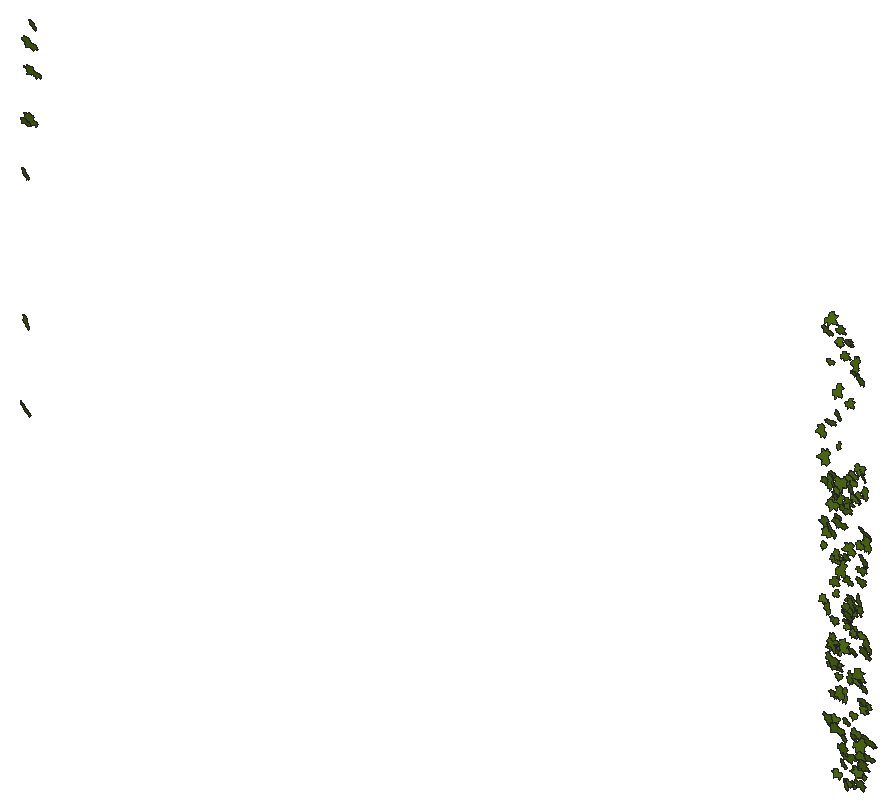
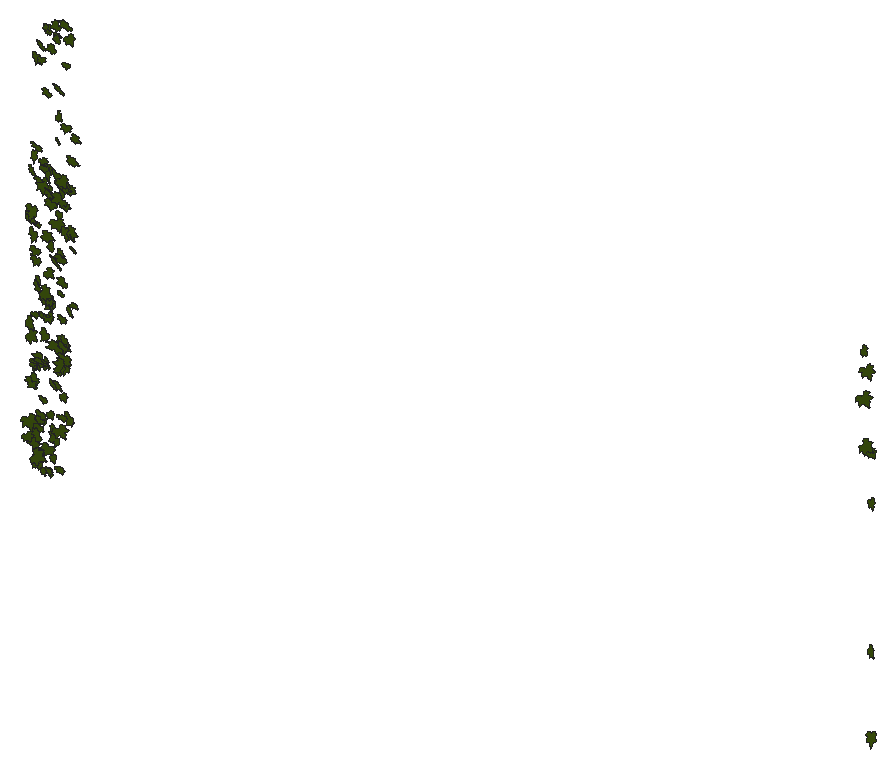
# SketchUp Ruby script. Lengths in inches.
U = 1.inch
M = Sketchup.active_model
def pt(a) = Geom::Point3d.new(a.map { |v| v * U })
def face(e, loops, mat)
  f = e.add_face(loops[0].map { |a| pt(a) })
  loops[1..].each { |l| e.add_face(l.map { |a| pt(a) }).erase! }
  f.material = f.back_material = mat if mat
  f
end
# faces: each face lists its corners as indices into pts; further lists are holes
def faces(e, pts, list, mat = nil) = list.each { |f| face(e, (f[0].is_a?(Array) ? f : [f]).map { |l| l.map { |i| pts[i] } }, mat) }
# xy, xz, yz: faces in a plane at the given z, y or x. An outline is a flat list of corners, or four numbers for a rectangle; further outlines are holes
def ring(l) = l.size == 4 ? [[l[0], l[1]], [l[2], l[1]], [l[2], l[3]], [l[0], l[3]]] : l.each_slice(2).to_a
def flat(e, list, mat, &to3) = list.each { |f| face(e, (f[0].is_a?(Array) ? f : [f]).map { |l| ring(l).map { |u, v| to3.(u, v) } }, mat) }
def xy(e, z, list, mat = nil) = flat(e, list, mat) { |x, y| [x, y, z] }
def xz(e, y, list, mat = nil) = flat(e, list, mat) { |x, z| [x, y, z] }
def yz(e, x, list, mat = nil) = flat(e, list, mat) { |y, z| [x, y, z] }
def lines(e, pts, list) = list.each { |a, b| e.add_line(pt(pts[a]), pt(pts[b])) }
# prism: a flat outline (further loops are holes) pulled along v
def prism(e, loops, v, mat = nil)
  f = face(e, loops, mat); d = Geom::Vector3d.new(v.map { |x| x * U })
  f.pushpull(f.normal.samedirection?(d) ? d.length : -d.length)
end
def box(e, o, s, mat = nil) = prism(e, [[o, [o[0] + s[0], o[1], o[2]], [o[0] + s[0], o[1] + s[1], o[2]], [o[0], o[1] + s[1], o[2]]]], [0, 0, s[2]], mat)
def at(x, y, z, deg = 0) = Geom::Transformation.translation(pt([x, y, z])) * Geom::Transformation.rotation(ORIGIN, Z_AXIS, deg.degrees)
def axes(o, x, y, z) = Geom::Transformation.new([*x, 0, *y, 0, *z, 0, *pt(o).to_a, 1])
def part(name) = M.definitions.add(name)
# library, detail: a bought-in or finely detailed component or shape, given as its bounding box
def library(name, o, s) = part(name).tap { |d| box(d.entities, o, s) }
def detail(e, o, s) = box(e.add_group.entities, o, s)
def put(e, d, t, mat = nil) = e.add_instance(d, t).tap { |i| i.material = mat if mat }
def group(e, t, mat = nil) = e.add_group.tap { |g| g.transformation = t; g.material = mat if mat }.entities
root = M.entities
M.materials.add("[Vegetation Blur 03]").color = [83, 114, 18]
c1 = part("ivy")
xy(c1.entities,0,[[0.782,0,0.786,0,0.787,0.005,0.789,0.009,0.821,0.072,0.875,0.147,1.001,0.272,1.073,0.331,1.137,0.363,1.178,0.379,1.223,0.384,1.272,0.383,1.311,0.374,1.36,0.355,1.399,0.334,1.491,0.285,1.541,0.244,1.583,0.199,1.617,0.15,1.64,0.128,1.662,0.115,1.717,0.105,1.745,0.093,1.784,0.054,1.819,0.057,1.854,0.064,1.882,0.075,1.896,0.074,1.91,0.071,1.937,0.063,1.964,0.053,1.99,0.038,2.016,0.015,2.034,0.002,2.04,0,2.038,0.003,2.036,0.007,2.033,0.038,2.036,0.068,2.045,0.1,2.055,0.116,2.064,0.123,2.077,0.129,2.088,0.129,2.106,0.132,2.118,0.13,2.179,0.132,2.207,0.133,2.225,0.133,2.242,0.138,2.22,0.162,2.207,0.186,2.206,0.213,2.212,0.236,2.228,0.262,2.247,0.274,2.298,0.283,2.355,0.294,2.37,0.296,2.376,0.295,2.377,0.3,2.377,0.303,2.385,0.329,2.411,0.37,2.426,0.392,2.449,0.407,2.511,0.426,2.561,0.444,2.619,0.466,2.589,0.469,2.561,0.476,2.501,0.5,2.449,0.516,2.424,0.523,2.401,0.535,2.377,0.556,2.372,0.568,2.36,0.575,2.268,0.586,2.225,0.592,2.207,0.599,2.194,0.61,2.143,0.65,2.13,0.664,2.122,0.682,2.123,0.7,2.13,0.719,2.148,0.75,2.17,0.781,2.195,0.807,2.221,0.828,2.284,0.874,2.291,0.88,2.288,0.887,2.276,0.9,2.267,0.916,2.265,0.933,2.273,0.967,2.292,1.002,2.313,1.03,2.334,1.054,2.348,1.067,2.358,1.074,2.363,1.076,2.362,1.081,2.35,1.094,2.347,1.11,2.35,1.143,2.359,1.18,2.385,1.254,2.415,1.324,2.448,1.393,2.45,1.4,2.446,1.398,2.44,1.394,2.427,1.383,2.402,1.36,2.376,1.339,2.345,1.324,2.305,1.309,2.282,1.303,2.273,1.306,2.245,1.294,2.212,1.287,2.187,1.291,2.163,1.301,2.142,1.316,2.134,1.327,2.124,1.325,2.09,1.292,2.053,1.259,2.014,1.234,1.973,1.215,1.954,1.21,1.931,1.208,1.909,1.212,1.893,1.22,1.879,1.233,1.872,1.248,1.867,1.281,1.864,1.319,1.821,1.258,1.773,1.197,1.726,1.141,1.698,1.121,1.679,1.116,1.666,1.117,1.647,1.122,1.632,1.129,1.62,1.141,1.617,1.154,1.617,1.219,1.621,1.254,1.623,1.268,1.623,1.281,1.618,1.314,1.606,1.346,1.603,1.375,1.607,1.403,1.603,1.467,1.599,1.499,1.605,1.525,1.614,1.552,1.629,1.577,1.635,1.589,1.629,1.587,1.618,1.582,1.596,1.566,1.581,1.556,1.568,1.552,1.557,1.55,1.545,1.553,1.531,1.562,1.522,1.572,1.504,1.591,1.486,1.611,1.474,1.631,1.457,1.666,1.455,1.684,1.457,1.698,1.452,1.715,1.444,1.728,1.424,1.754,1.419,1.772,1.423,1.786,1.434,1.819,1.444,1.848,1.446,1.855,1.44,1.861,1.43,1.867,1.386,1.904,1.349,1.948,1.326,1.973,1.31,1.995,1.288,2.048,1.284,2.153,1.287,2.254,1.284,2.255,1.282,2.253,1.278,2.247,1.274,2.237,1.266,2.216,1.226,2.125,1.208,2.076,1.184,2.033,1.155,1.984,1.135,1.942,1.111,1.899,1.083,1.861,1.053,1.85,1.059,1.83,1.061,1.809,1.056,1.79,1.049,1.767,1.04,1.749,1.018,1.733,0.994,1.726,0.942,1.734,0.95,1.6875,0.944,1.645,0.932,1.608,0.911,1.585,0.881,1.58,0.854,1.582,0.828,1.588,0.785,1.618,0.773,1.625,0.775,1.614,0.779,1.598,0.796,1.502,0.818,1.402,0.861,1.283,0.882,1.224,0.894,1.174,0.892,1.148,0.886,1.123,0.881,1.107,0.872,1.099,0.849,1.094,0.818,1.092,0.789,1.098,0.762,1.107,0.753,1.113,0.721,1.139,0.698,1.163,0.678,1.194,0.665,1.224,0.628,1.28,0.612,1.312,0.606,1.327,0.606,1.314,0.599,1.282,0.594,1.267,0.581,1.256,0.544,1.245,0.512,1.244,0.473,1.249,0.444,1.256,0.382,1.288,0.339,1.306,0.324,1.316,0.317,1.324,0.309,1.326,0.27,1.314,0.227,1.313,0.185,1.3125,0.152,1.317,0.122,1.328,0.092,1.345,0.073,1.353,0.079,1.338,0.092,1.308,0.117,1.249,0.13,1.215,0.139,1.164,0.147,1.148,0.157,1.136,0.163,1.122,0.174,1.086,0.177,1.067,0.182,1.054,0.186,1.043,0.191,1.038,0.211,1.028,0.237,1.005,0.25,0.974,0.253,0.96,0.25,0.944,0.242,0.914,0.243,0.906,0.249,0.902,0.26,0.894,0.289,0.88,0.307,0.873,0.322,0.862,0.364,0.799,0.403,0.738,0.431,0.709,0.439,0.691,0.441,0.678,0.4375,0.66,0.428,0.645,0.394,0.623,0.303,0.594,0.255,0.581,0.214,0.577,0.179,0.573,0.173,0.568,0.175,0.561,0.167,0.55,0.141,0.523,0.113,0.503,0.077,0.49,0.045,0.486,0.026,0.485,0.019,0.486,0.011,0.483,0,0.471,0.014,0.467,0.044,0.455,0.058,0.447,0.07,0.438,0.097,0.411,0.125,0.394,0.158,0.377,0.174,0.366,0.182,0.359,0.185,0.361,0.242,0.331,0.253,0.316,0.258,0.303,0.262,0.283,0.274,0.278,0.308,0.274,0.341,0.252,0.366,0.226,0.366,0.222,0.37,0.22,0.38,0.221,0.395,0.221,0.425,0.216,0.45,0.207,0.465,0.192,0.473,0.178,0.484,0.15,0.489,0.116,0.483,0.089,0.468,0.058,0.45,0.035,0.435,0.018,0.429,0.011,0.434,0.012,0.438,0.014,0.469,0.019,0.542,0.016,0.581,0.015,0.612,0.027,0.68,0.055,0.696,0.057,0.712,0.052,0.73,0.045,0.741,0.036,0.766,0.014]])
p = [[34,174,142.56],[33.92,174,142.56]]
lines(root,p,[[0,1]])
put(root,c1,axes([31.04,173.2,134.52],[0.25146,0.10077,-0.27244],[-0.33679,0.12568,-0.19974],[-0.01997,-0.85077,-0.06178]),"[Vegetation Blur 03]")
put(root,c1,axes([31.31,173.2,115.84],[0.20676,-0.07941,-0.38547],[-0.44776,0.31453,-0.17016],[-0.15519,-1.01328,-0.02261]),"[Vegetation Blur 03]")
put(root,c1,axes([31.04,173.2,129.8],[0.3273,-0.0909,-0.29956],[-0.34726,0.27044,-0.26563],[-0.12681,-0.97518,-0.04574]),"[Vegetation Blur 03]")
put(root,c1,axes([30.73,173.2,107.71],[0.5589,-0.19272,-0.25961],[-0.28238,0.39595,-0.45114],[-0.17385,-1.26271,-0.10184]),"[Vegetation Blur 03]")
put(root,c1,axes([31.24,173.2,142.33],[0.49914,0.06889,-0.35402],[-0.43405,0.1716,-0.40237],[-0.0297,-1.34994,-0.06922]),"[Vegetation Blur 03]")
put(root,c1,axes([31.88,173.2,135.19],[0.20681,0.14961,-0.50522],[-0.62308,0.08477,-0.16594],[-0.01632,-1.34039,-0.06689]),"[Vegetation Blur 03]")
put(root,c1,axes([31.61,173.2,139.73],[0.44413,0.17265,-0.41061],[-0.51006,0.15289,-0.35736],[-0.00095,-1.3725,-0.09146]),"[Vegetation Blur 03]")
put(root,c1,axes([31.96,173.2,143.91],[0.1485,0.06744,-0.32773],[-0.39216,0.22625,-0.11103],[-0.09244,-0.8515,-0.05546]),"[Vegetation Blur 03]")
put(root,c1,axes([114.99,173.7,134.86],[0.22705,-0.11945,-0.35491],[-0.43835,-0.02,-0.18572],[-0.01818,-1.0093,0.04569]),"[Vegetation Blur 03]")
put(root,c1,axes([115.44,173.7,126.11],[0.07342,0.0201,-0.45241],[-0.55143,0.12193,-0.05876],[-0.05747,-1.14418,-0.01421]),"[Vegetation Blur 03]")
put(root,c1,axes([115,173.7,118.84],[0.22258,-0.06561,-0.19839],[-0.24493,-0.08915,-0.17839],[0.01076,-0.67235,0.04301]),"[Vegetation Blur 03]")
put(root,c1,axes([115.28,173.7,129.93],[0.13601,0.05917,-0.30855],[-0.37908,0.03752,-0.11017],[-0.00748,-0.82593,-0.02711]),"[Vegetation Blur 03]")
put(root,c1,axes([115.11,173.7,144.26],[0.33145,0.05992,-0.29685],[-0.36343,0.14447,-0.2657],[-0.03257,-1.00226,-0.05605]),"[Vegetation Blur 03]")
put(root,c1,axes([115.64,173.7,132.65],[0.1603,-0.20672,-0.46475],[-0.57787,-0.01388,-0.13179],[-0.02063,-1.21728,0.08043]),"[Vegetation Blur 03]")
put(root,c1,axes([114.82,173.7,123.76],[0.29106,-0.10296,0.03164],[0.02588,-0.14904,-0.23485],[-0.05776,-0.58557,0.05421]),"[Vegetation Blur 03]")
put(root,c1,axes([115.22,173.7,125.33],[0.3254,-0.08509,-0.21734],[-0.269,-0.05049,-0.26515],[-0.01633,-0.86378,0.03691]),"[Vegetation Blur 03]")
put(root,c1,axes([115.52,173.7,118.41],[0.27571,-0.25978,-0.33675],[-0.40528,0.18997,-0.24407],[-0.14812,-1.00337,0.04098]),"[Vegetation Blur 03]")
put(root,c1,axes([115.87,173.7,130.26],[0.12192,-0.00071,-0.41999],[-0.49465,0.29998,-0.09572],[-0.14193,-1.04612,-0.02717]),"[Vegetation Blur 03]")
put(root,c1,axes([115.9,173.7,130.28],[0.14174,-0.20689,-0.42841],[-0.51411,0.25268,-0.13249],[-0.14609,-1.08996,0.0506]),"[Vegetation Blur 03]")
put(root,c1,axes([115.13,173.7,135.43],[0.38883,0.03177,-0.00541],[-0.00902,0.12865,-0.31342],[0.01417,-0.78985,-0.05127]),"[Vegetation Blur 03]")
put(root,c1,axes([115.375,173.7,141.22],[0.29737,0.00668,-0.03254],[-0.03987,-0.00069,-0.24271],[0.00326,-0.6174,-0.00008]),"[Vegetation Blur 03]")
put(root,c1,axes([115.875,173.7,114.67],[0.1748,-0.10036,-0.26156],[-0.32362,-0.01023,-0.14344],[-0.01895,-0.75115,0.0369]),"[Vegetation Blur 03]")
put(root,c1,axes([114.85,173.7,107.66],[0.54065,-0.21536,0.14176],[0.17436,-0.02611,-0.44914],[-0.10356,-1.16826,-0.01609]),"[Vegetation Blur 03]")
put(root,c1,axes([114.91,173.7,144.53],[0.22945,0.18892,0.3925],[0.48869,-0.02142,-0.18866],[0.02999,-1.09631,0.07132]),"[Vegetation Blur 03]")
put(root,c1,axes([115.86,173.7,130.72],[0.32489,0.11128,-0.34401],[-0.42351,0.17483,-0.25752],[-0.03505,-1.08109,-0.07706]),"[Vegetation Blur 03]")
put(root,c1,axes([115.32,173.7,125.73],[0.57169,-0.21875,-0.18427],[-0.21197,0.1873,-0.473],[-0.13171,-1.2509,-0.0386]),"[Vegetation Blur 03]")
put(root,c1,axes([115.83,173.7,110.08],[0.26898,-0.00531,-0.22272],[-0.27011,0.10743,-0.21769],[-0.03898,-0.78115,-0.02842]),"[Vegetation Blur 03]")
put(root,c1,axes([116.15,173.7,115.51],[0.26861,-0.16753,-0.42435],[-0.51691,0.14174,-0.22674],[-0.09889,-1.19591,0.03257]),"[Vegetation Blur 03]")
put(root,c1,axes([115.5,173.7,128.02],[0.48108,0.0091,-0.09014],[-0.10924,-0.11608,-0.39016],[0.0169,-1.00907,0.04407]),"[Vegetation Blur 03]")
put(root,c1,axes([115.25,173.7,113.55],[0.65346,-0.15996,-0.07236],[-0.08578,0.05992,-0.53686],[-0.0809,-1.3557,-0.01519]),"[Vegetation Blur 03]")
put(root,c1,axes([115.96,173.7,107.125],[0.44397,0.1395,-0.34863],[-0.43136,0.05055,-0.3627],[0.03168,-1.26682,-0.05286]),"[Vegetation Blur 03]")
put(root,c1,axes([115.92,173.7,112.72],[0.30297,0.01543,-0.16149],[-0.19571,0.1367,-0.2425],[-0.03016,-0.73198,-0.04869]),"[Vegetation Blur 03]")
put(root,c1,axes([115.91,173.7,107.875],[0.36198,-0.00364,-0.10329],[-0.12566,-0.10485,-0.29275],[0.01516,-0.7821,0.03972]),"[Vegetation Blur 03]")
put(root,c1,axes([116.55,173.7,136.52],[0.10541,0.02404,-0.33372],[-0.3979,0.2077,-0.08136],[-0.09494,-0.84377,-0.02954]),"[Vegetation Blur 03]")
put(root,c1,axes([115.51,173.7,120.11],[0.22933,0.01454,0.32661],[0.40022,0.004,-0.18721],[0.0052,-0.94915,0.00421]),"[Vegetation Blur 03]")
put(root,c1,axes([115.6875,173.7,117.01],[0.4011,-0.07198,0.04538],[0.05521,-0.01426,-0.32859],[-0.0356,-0.83315,0.0017]),"[Vegetation Blur 03]")
put(root,c1,axes([115.85,173.7,128.88],[0.3582,-0.18702,-0.03708],[-0.03384,0.10347,-0.29982],[-0.09581,-0.73577,-0.03274]),"[Vegetation Blur 03]")
put(root,c1,axes([115.33,173.7,114.79],[0.61675,-0.12461,0.11294],[0.13479,-0.08629,-0.50526],[-0.06818,-1.29784,0.02275]),"[Vegetation Blur 03]")
put(root,c1,axes([115.16,173.7,112.34],[0.50593,-0.03643,0.3437],[0.41936,0.17969,-0.40818],[0.0424,-1.34262,-0.06395]),"[Vegetation Blur 03]")
put(root,c1,axes([116.57,173.7,123.52],[0.12968,-0.11784,-0.31424],[-0.38451,0.09135,-0.11108],[-0.06065,-0.83104,0.03235]),"[Vegetation Blur 03]")
put(root,c1,axes([115.5,173.7,114.26],[0.44883,-0.14962,0.17944],[0.22549,0.05754,-0.36812],[-0.05276,-1.02686,-0.04677]),"[Vegetation Blur 03]")
put(root,c1,axes([115.86,173.7,119.08],[0.14273,0.06127,0.20808],[0.25666,-0.04237,-0.11531],[-0.00355,-0.59977,0.0294]),"[Vegetation Blur 03]")
put(root,c1,axes([115.56,173.7,122.49],[0.3729,0.07352,0.23123],[0.28448,-0.01242,-0.30497],[0.02479,-0.96364,0.02157]),"[Vegetation Blur 03]")
put(root,c1,axes([116.125,173.7,126.48],[0.49872,0.09657,-0.2358],[-0.29251,0.12066,-0.4043],[0.0109,-1.17989,-0.06065]),"[Vegetation Blur 03]")
put(root,c1,axes([116.25,173.7,102.9],[0.37574,-0.07096,-0.15978],[-0.19839,-0.07956,-0.3052],[-0.01253,-0.86822,0.04103]),"[Vegetation Blur 03]")
put(root,c1,axes([116.11,173.7,126.86],[0.33145,-0.08577,-0.02014],[-0.01771,0.11215,-0.26935],[-0.04508,-0.6747,-0.04221]),"[Vegetation Blur 03]")
put(root,c1,axes([115.47,173.7,127.82],[0.38163,0.10723,0.44815],[0.5511,-0.01709,-0.31195],[0.0229,-1.37595,0.0388]),"[Vegetation Blur 03]")
put(root,c1,axes([115.79,173.7,138.07],[0.21319,0.1755,0.40106],[0.49372,-0.23014,-0.15897],[-0.07069,-1.078,0.09923]),"[Vegetation Blur 03]")
put(root,c1,axes([116.23,173.7,111.84],[0.32221,-0.0387,0.02273],[0.02664,-0.04287,-0.26295],[-0.0205,-0.66413,0.01565]),"[Vegetation Blur 03]")
put(root,c1,axes([116.03,173.7,129.23],[0.32579,-0.0019,0.20222],[0.24053,-0.19974,-0.25841],[-0.05947,-0.81825,0.06261]),"[Vegetation Blur 03]")
put(root,c1,axes([116.35,173.7,133.17],[0.07732,0.04701,0.24249],[0.28519,-0.19481,-0.05463],[-0.0864,-0.60099,0.03668]),"[Vegetation Blur 03]")
put(root,c1,axes([117.03,173.7,143.72],[0.09099,-0.0894,-0.27257],[-0.33609,-0.07013,-0.07111],[0.02177,-0.70885,0.04141]),"[Vegetation Blur 03]")
put(root,c1,axes([116.31,173.7,142.77],[0.07701,-0.01607,0.28736],[0.35217,-0.0014,-0.06288],[-0.00233,-0.74167,-0.00611]),"[Vegetation Blur 03]")
put(root,c1,axes([116.86,173.7,110.86],[0.33179,-0.22508,-0.3253],[-0.40723,0.00189,-0.27687],[-0.0707,-1.0672,0.06812]),"[Vegetation Blur 03]")
put(root,c1,axes([115.87,173.7,113.75],[0.25598,0.2014,0.48378],[0.59803,0.04143,-0.21349],[0.05748,-1.32803,0.06671]),"[Vegetation Blur 03]")
put(root,c1,axes([116.18,173.7,144.13],[0.23882,-0.04134,0.29544],[0.36225,0.06442,-0.19363],[0.01513,-0.89011,-0.02773]),"[Vegetation Blur 03]")
put(root,c1,axes([116.87,173.7,103.89],[0.29522,-0.08617,-0.18688],[-0.21829,0.16177,-0.24143],[-0.08083,-0.75161,-0.03054]),"[Vegetation Blur 03]")
put(root,c1,axes([116.125,173.7,130.33],[0.60257,-0.08021,0.1387],[0.16152,-0.21723,-0.48713],[-0.06569,-1.26991,0.07457]),"[Vegetation Blur 03]")
put(root,c1,axes([116.16,173.7,121.39],[0.26041,0.16269,0.49935],[0.59768,-0.40532,-0.18684],[-0.15294,-1.30696,0.1201]),"[Vegetation Blur 03]")
put(root,c1,axes([116.62,173.7,127.86],[0.50551,0.02715,-0.04471],[-0.05585,0.1053,-0.41049],[0.00753,-1.04102,-0.04269]),"[Vegetation Blur 03]")
put(root,c1,axes([117.2,173.7,107.91],[0.2455,0.02361,-0.20397],[-0.24867,0.10235,-0.19749],[-0.02754,-0.71362,-0.03507]),"[Vegetation Blur 03]")
put(root,c1,axes([117.43,173.7,110.82],[0.25932,-0.29593,-0.35358],[-0.43934,0.11655,-0.22996],[-0.12392,-1.03246,0.07539]),"[Vegetation Blur 03]")
put(root,c1,axes([117.24,173.7,118.6],[0.23892,0.03876,-0.2007],[-0.24369,0.14566,-0.1888],[-0.038,-0.69034,-0.0511]),"[Vegetation Blur 03]")
put(root,c1,axes([117.51,173.7,121.42],[0.22065,0.07279,-0.34055],[-0.41864,0.06201,-0.17859],[-0.01021,-0.96933,-0.037]),"[Vegetation Blur 03]")
put(root,c1,axes([116.6875,173.7,141.74],[0.16739,0.00231,0.3142],[0.38437,0.04772,-0.13645],[0.02172,-0.86254,-0.00671]),"[Vegetation Blur 03]")
put(root,c1,axes([117.25,173.7,117.24],[0.33471,0.047,-0.24757],[-0.30145,0.17573,-0.26622],[-0.0408,-0.91277,-0.064]),"[Vegetation Blur 03]")
put(root,c1,axes([116.79,173.7,106.03],[0.27088,-0.15261,0.15464],[0.19269,-0.01614,-0.22733],[-0.06536,-0.68006,-0.0293]),"[Vegetation Blur 03]")
put(root,c1,axes([116.33,173.7,105.01],[0.44693,-0.21309,0.34937],[0.42945,-0.06761,-0.37241],[-0.09772,-1.27172,-0.03874]),"[Vegetation Blur 03]")
put(root,c1,axes([117.03,173.7,116.37],[0.12441,0.10653,0.22366],[0.27873,-0.02631,-0.1013],[0.00957,-0.61876,0.04281]),"[Vegetation Blur 03]")
put(root,c1,axes([117.2,173.7,102.22],[0.37274,-0.27698,-0.10257],[-0.11734,0.09274,-0.32343],[-0.14192,-0.80413,-0.00197]),"[Vegetation Blur 03]")
put(root,c1,axes([118.15,173.7,119.6],[0.10808,0.0782,-0.51354],[-0.62715,0.14615,-0.08441],[-0.06373,-1.30565,-0.04021]),"[Vegetation Blur 03]")
put(root,c1,axes([117.03,173.7,122.97],[0.1451,-0.1312,0.25798],[0.3214,0.00081,-0.12034],[-0.02623,-0.71573,-0.04743]),"[Vegetation Blur 03]")
put(root,c1,axes([117,173.7,128.03],[0.20968,0.01131,0.23173],[0.28004,-0.12895,-0.16779],[-0.0472,-0.71481,0.03394]),"[Vegetation Blur 03]")
put(root,c1,axes([117.25,173.7,118.875],[0.56655,-0.0115,-0.27779],[-0.34007,0.04247,-0.46224],[-0.01542,-1.35941,-0.01209]),"[Vegetation Blur 03]")
put(root,c1,axes([117.58,173.7,130.89],[0.41729,-0.27977,-0.39423],[-0.44817,0.37379,-0.3577],[-0.22574,-1.25924,-0.01859]),"[Vegetation Blur 03]")
put(root,c1,axes([116.79,173.7,104.41],[0.53014,0.02962,0.10212],[0.12282,0.12551,-0.4304],[0.02794,-1.11386,-0.04578]),"[Vegetation Blur 03]")
put(root,c1,axes([117.9375,173.7,119.35],[0.21226,-0.08156,-0.39258],[-0.47103,0.20087,-0.17619],[-0.10528,-1.06312,-0.00317]),"[Vegetation Blur 03]")
put(root,c1,axes([118.07,173.7,124.72],[0.17219,-0.03701,-0.43547],[-0.53302,-0.07752,-0.13935],[0.03036,-1.15115,0.02338]),"[Vegetation Blur 03]")
put(root,c1,axes([117.32,173.7,102.29],[0.37414,-0.10141,-0.07585],[-0.09511,-0.0243,-0.3074],[-0.04493,-0.79294,0.01912]),"[Vegetation Blur 03]")
put(root,c1,axes([116.73,173.7,117.96],[0.55336,-0.2755,0.17895],[0.23761,0.14136,-0.45516],[-0.0977,-1.21665,-0.0934]),"[Vegetation Blur 03]")
put(root,c1,axes([117,173.7,127.98],[0.16066,-0.07376,0.37357],[0.45903,0.04715,-0.13002],[0.00982,-0.99714,-0.03378]),"[Vegetation Blur 03]")
put(root,c1,axes([117.67,173.7,131.1],[0.38856,-0.00058,-0.29483],[-0.35992,-0.09405,-0.31593],[0.03091,-1.0877,0.02748]),"[Vegetation Blur 03]")
put(root,c1,axes([117.25,173.7,143.37],[0.16816,-0.15089,0.24654],[0.3088,-0.00002,-0.1403],[-0.03567,-0.71145,-0.05229]),"[Vegetation Blur 03]")
put(root,c1,axes([117.15,173.7,137.5],[0.24024,0.06291,0.29442],[0.3619,-0.06648,-0.19446],[-0.01006,-0.88941,0.03536]),"[Vegetation Blur 03]")
put(root,c1,axes([117.48,173.7,117.9],[0.13772,-0.02232,0.26418],[0.31478,-0.16115,-0.11144],[-0.07624,-0.70573,0.01709]),"[Vegetation Blur 03]")
put(root,c1,axes([117.7,173.7,129.74],[0.55985,-0.09656,-0.30764],[-0.35518,0.35678,-0.44814],[-0.13469,-1.34226,-0.09699]),"[Vegetation Blur 03]")
put(root,c1,axes([117.42,173.7,111.54],[0.07106,0.03212,0.39333],[0.4647,-0.27217,-0.05243],[-0.12873,-0.96482,0.02788]),"[Vegetation Blur 03]")
put(root,c1,axes([118.01,173.7,102.25],[0.22842,-0.06235,-0.19773],[-0.23665,0.11144,-0.18763],[-0.06007,-0.67607,-0.01269]),"[Vegetation Blur 03]")
put(root,c1,axes([117.92,173.7,131.52],[0.31144,-0.00755,-0.1936],[-0.23722,0.00118,-0.25419],[-0.00327,-0.80561,0.00144]),"[Vegetation Blur 03]")
put(root,c1,axes([117.54,173.7,143.37],[0.14289,-0.07488,0.25812],[0.31299,-0.09737,-0.11985],[-0.0582,-0.70749,-0.01082]),"[Vegetation Blur 03]")
put(root,c1,axes([117.89,173.7,140.96],[0.30877,0.02964,-0.06253],[-0.07793,0.09874,-0.24894],[0.00225,-0.64717,-0.04084]),"[Vegetation Blur 03]")
put(root,c1,axes([117.43,173.7,114.76],[0.46892,-0.24319,0.11777],[0.16224,0.13537,-0.38629],[-0.09203,-1.00049,-0.08089]),"[Vegetation Blur 03]")
put(root,c1,axes([117.76,173.7,108.71],[0.35341,-0.05372,0.02619],[0.03014,-0.05475,-0.28854],[-0.02834,-0.72817,0.01976]),"[Vegetation Blur 03]")
put(root,c1,axes([117.98,173.7,116.64],[0.31975,-0.13436,-0.03342],[-0.05173,-0.10756,-0.26163],[-0.05713,-0.65457,0.04985]),"[Vegetation Blur 03]")
put(root,c1,axes([117.79,173.7,106.5],[0.29444,-0.13699,0.14225],[0.1786,0.0132,-0.24425],[-0.05394,-0.70397,-0.03226]),"[Vegetation Blur 03]")
put(root,c1,axes([117.7,173.7,116.09],[0.20883,0.04815,0.31421],[0.37772,-0.20796,-0.1622],[-0.0781,-0.87697,0.05572]),"[Vegetation Blur 03]")
put(root,c1,axes([119.03,173.7,103.86],[0.10967,0.16764,-0.53959],[-0.66571,-0.0227,-0.09123],[0.02429,-1.37893,-0.0641]),"[Vegetation Blur 03]")
put(root,c1,axes([118.83,173.7,142.43],[0.1383,-0.27518,-0.42018],[-0.52123,0.14835,-0.12955],[-0.10615,-1.08693,0.0887]),"[Vegetation Blur 03]")
put(root,c1,axes([117.5,173.7,111.87],[0.43423,0.11965,0.28912],[0.35873,-0.10053,-0.35232],[0.01383,-1.14881,0.06094]),"[Vegetation Blur 03]")
put(root,c1,axes([117.73,173.7,128.98],[0.34318,0.09184,0.26358],[0.326,-0.10859,-0.27677],[-0.00403,-0.96364,0.05631]),"[Vegetation Blur 03]")
put(root,c1,axes([117.97,173.7,107.3],[0.4987,-0.12613,-0.04723],[-0.0598,-0.02572,-0.40975],[-0.05942,-1.03278,0.01597]),"[Vegetation Blur 03]")
put(root,c1,axes([117.99,173.7,106.47],[0.24944,0.02336,0.19362],[0.23616,0.05082,-0.20362],[0.02524,-0.70655,-0.00824]),"[Vegetation Blur 03]")
put(root,c1,axes([118.67,173.7,111.9],[0.17883,0.01791,-0.19414],[-0.23754,0.05276,-0.14498],[-0.01529,-0.61012,-0.01823]),"[Vegetation Blur 03]")
put(root,c1,axes([117.57,173.7,111.91],[0.34678,0.03788,0.46084],[0.56412,0.05104,-0.28341],[0.03077,-1.36263,0.00219]),"[Vegetation Blur 03]")
put(root,c1,axes([118.625,173.7,120.12],[0.31941,-0.24553,-0.21108],[-0.24847,0.1507,-0.27802],[-0.13923,-0.8322,0.01193]),"[Vegetation Blur 03]")
put(root,c1,axes([118.19,173.7,103.7],[0.48615,-0.06506,-0.03255],[-0.04363,-0.12709,-0.39413],[-0.0262,-0.99568,0.05243]),"[Vegetation Blur 03]")
put(root,c1,axes([118.68,173.7,125.18],[0.29981,-0.06525,-0.13535],[-0.1686,-0.07812,-0.24283],[-0.00912,-0.70071,0.03968]),"[Vegetation Blur 03]")
put(root,c1,axes([119.36,173.7,115.15],[0.17288,0.13727,-0.46997],[-0.57483,0.20036,-0.13164],[-0.0749,-1.22089,-0.07445]),"[Vegetation Blur 03]")
put(root,c1,axes([118.38,173.7,122.55],[0.40772,-0.01716,0.08723],[0.10718,0.04684,-0.33224],[-0.00228,-0.8661,-0.01969]),"[Vegetation Blur 03]")
put(root,c1,axes([118.82,173.7,116.62],[0.28445,-0.01133,-0.1134],[-0.139,-0.04223,-0.23156],[0.00407,-0.65007,0.01702]),"[Vegetation Blur 03]")
put(root,c1,axes([118.75,173.7,131.88],[0.40706,-0.21039,-0.21028],[-0.21941,0.3311,-0.33502],[-0.1694,-0.93442,-0.07136]),"[Vegetation Blur 03]")
put(root,c1,axes([118.34,173.7,132.3125],[0.49447,-0.06651,0.04707],[0.05156,-0.17262,-0.39913],[-0.04138,-1.00977,0.06513]),"[Vegetation Blur 03]")
put(root,c1,axes([118.41,173.7,140.84],[0.50217,-0.23211,-0.02067],[-0.01614,0.08923,-0.41886],[-0.11447,-1.03084,-0.03161]),"[Vegetation Blur 03]")
put(root,c1,axes([117.95,173.7,105.65],[0.43574,0.04341,0.40329],[0.4922,-0.17124,-0.35133],[-0.04861,-1.34487,0.05775]),"[Vegetation Blur 03]")
put(root,c1,axes([118.26,173.7,104.53],[0.18345,-0.01602,0.41607],[0.50825,-0.08298,-0.14976],[-0.04057,-1.11184,0.00518]),"[Vegetation Blur 03]")
put(root,c1,axes([118.16,173.7,102.36],[0.49317,-0.18476,0.20262],[0.2548,0.0498,-0.40595],[-0.06909,-1.1351,-0.05079]),"[Vegetation Blur 03]")
put(root,c1,axes([118.34,173.7,121.625],[0.48848,-0.12647,0.08295],[0.10536,0.05262,-0.40062],[-0.05484,-1.02537,-0.03079]),"[Vegetation Blur 03]")
put(root,c1,axes([118.38,173.7,118.84],[0.37427,-0.16845,0.18276],[0.21743,-0.11081,-0.31265],[-0.09784,-0.89065,0.00433]),"[Vegetation Blur 03]")
put(root,c1,axes([118.75,173.7,111.94],[0.464,-0.18688,-0.09777],[-0.10719,0.14954,-0.38378],[-0.10541,-0.97473,-0.04013]),"[Vegetation Blur 03]")
put(root,c1,axes([118.52,173.7,110.15],[0.36419,-0.14328,0.1768],[0.2225,0.04791,-0.29916],[-0.04769,-0.87068,-0.04556]),"[Vegetation Blur 03]")
put(root,c1,axes([119.61,173.7,130.38],[0.12813,-0.15006,-0.36786],[-0.44192,0.20151,-0.11546],[-0.11482,-0.94298,0.03387]),"[Vegetation Blur 03]")
put(root,c1,axes([119.06,173.7,107.03],[0.53027,0.09687,-0.32245],[-0.39653,0.24084,-0.42296],[-0.03295,-1.33931,-0.09938]),"[Vegetation Blur 03]")
put(root,c1,axes([118.68,173.7,126.54],[0.61753,-0.18671,-0.12394],[-0.12621,0.33022,-0.49708],[-0.12397,-1.26626,-0.11135]),"[Vegetation Blur 03]")
put(root,c1,axes([119.63,173.7,116.17],[0.24952,-0.09563,-0.45788],[-0.54485,0.27669,-0.20686],[-0.14163,-1.23287,-0.01091]),"[Vegetation Blur 03]")
put(root,c1,axes([118.48,173.7,103.85],[0.29611,-0.16504,0.41768],[0.51687,0.01316,-0.24325],[-0.03458,-1.21665,-0.05929]),"[Vegetation Blur 03]")
put(root,c1,axes([118.76,173.7,109.44],[0.29238,-0.00543,0.2431],[0.28843,-0.20948,-0.23179],[-0.07444,-0.83296,0.05671]),"[Vegetation Blur 03]")
put(root,c1,axes([118.71,173.7,123.97],[0.56984,-0.3114,0.00181],[0.01697,0.11385,-0.47886],[-0.15039,-1.16708,-0.04719]),"[Vegetation Blur 03]")
put(root,c1,axes([119.42,173.7,105.23],[0.30579,0.15468,-0.23311],[-0.2938,0.07258,-0.24913],[0.03027,-0.858,-0.0631]),"[Vegetation Blur 03]")
put(root,c1,axes([119.89,173.7,125.98],[0.21628,-0.19716,-0.4852],[-0.59473,0.13393,-0.18514],[-0.09444,-1.29492,0.05473]),"[Vegetation Blur 03]")
put(root,c1,axes([118.71,173.7,109.84],[0.46672,-0.03992,0.15461],[0.18977,0.01161,-0.3811],[-0.01585,-1.03645,-0.01022]),"[Vegetation Blur 03]")
